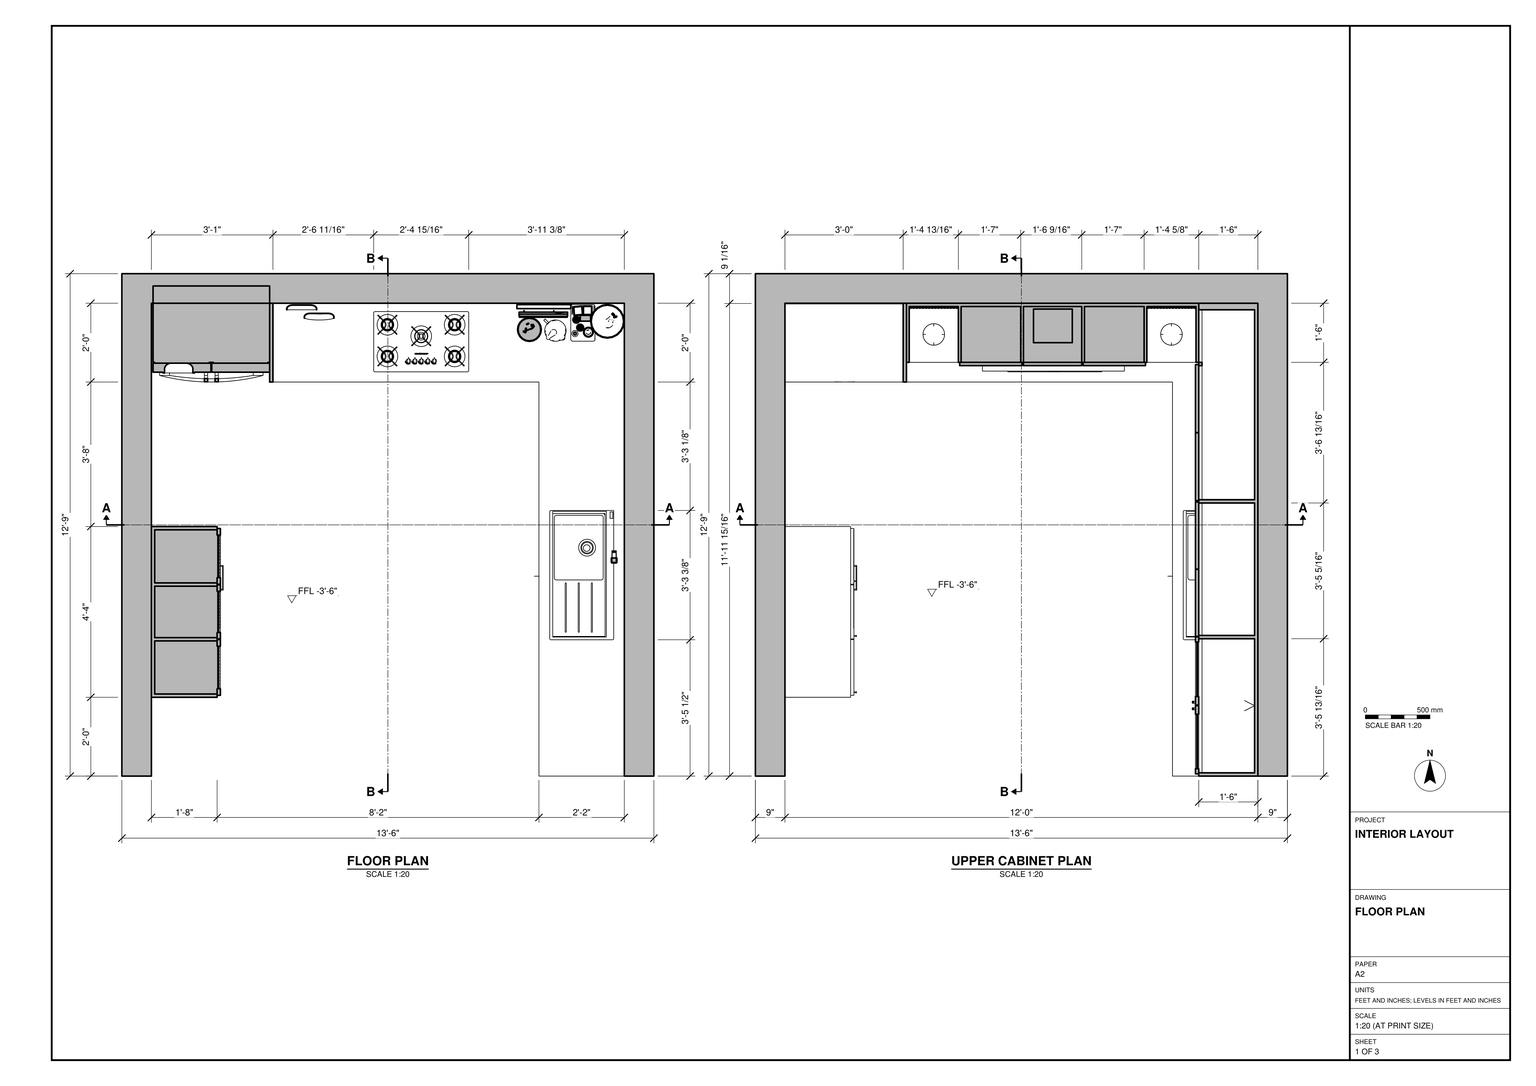
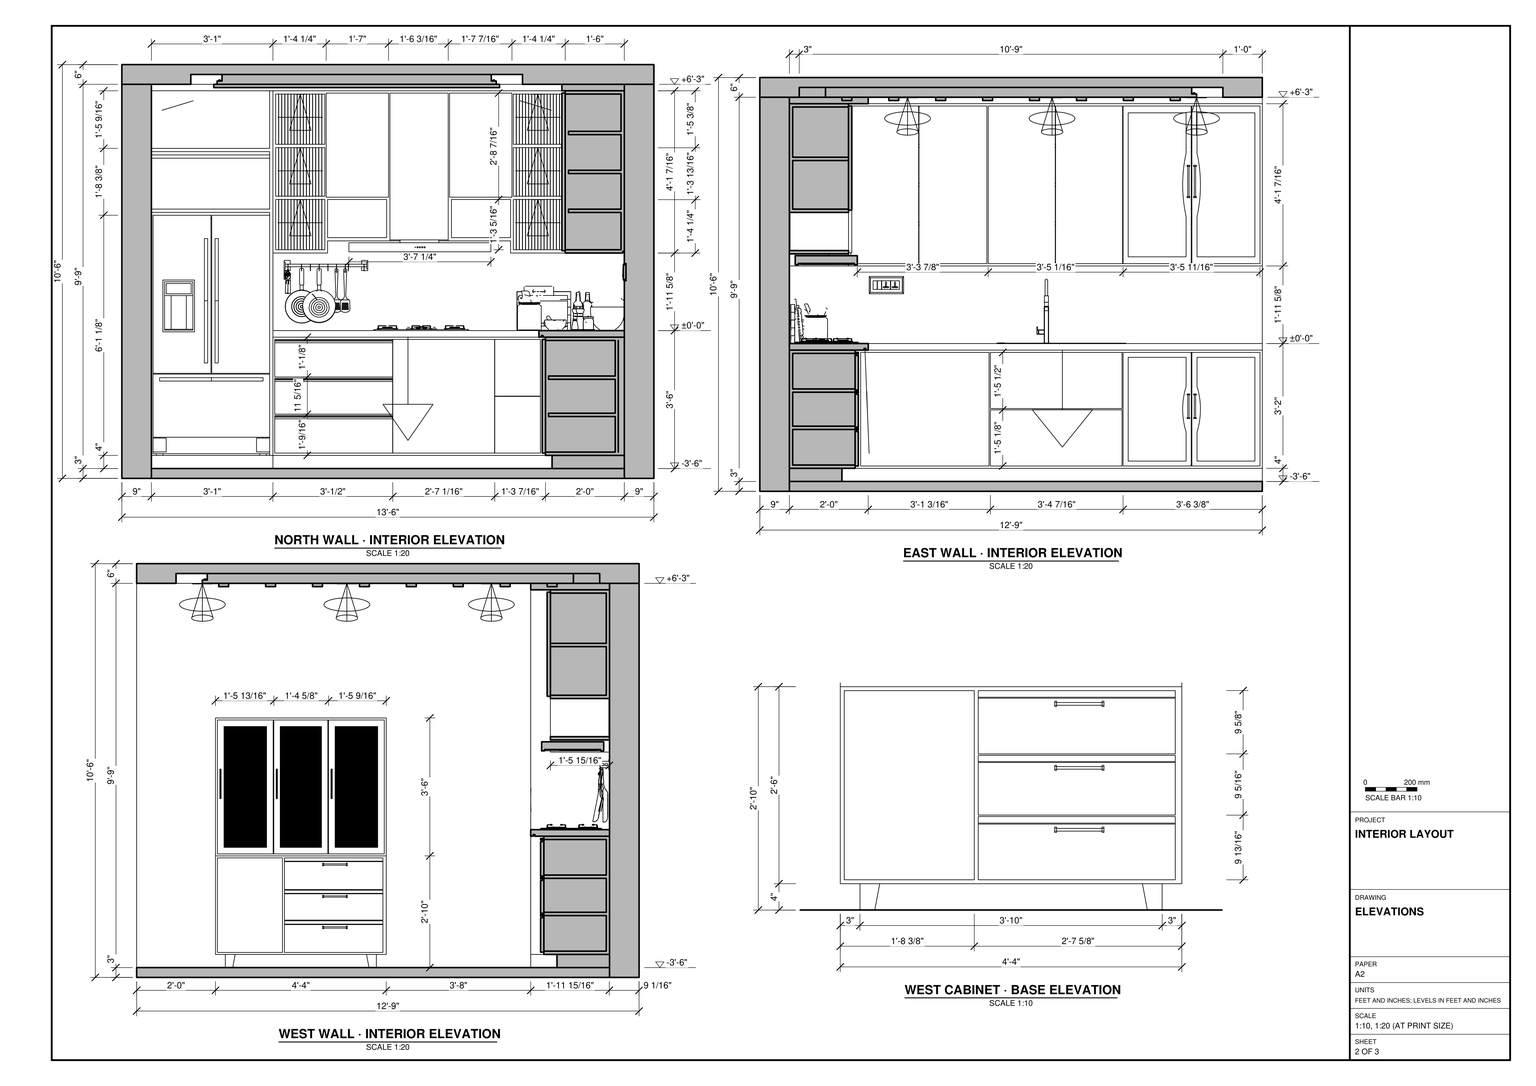
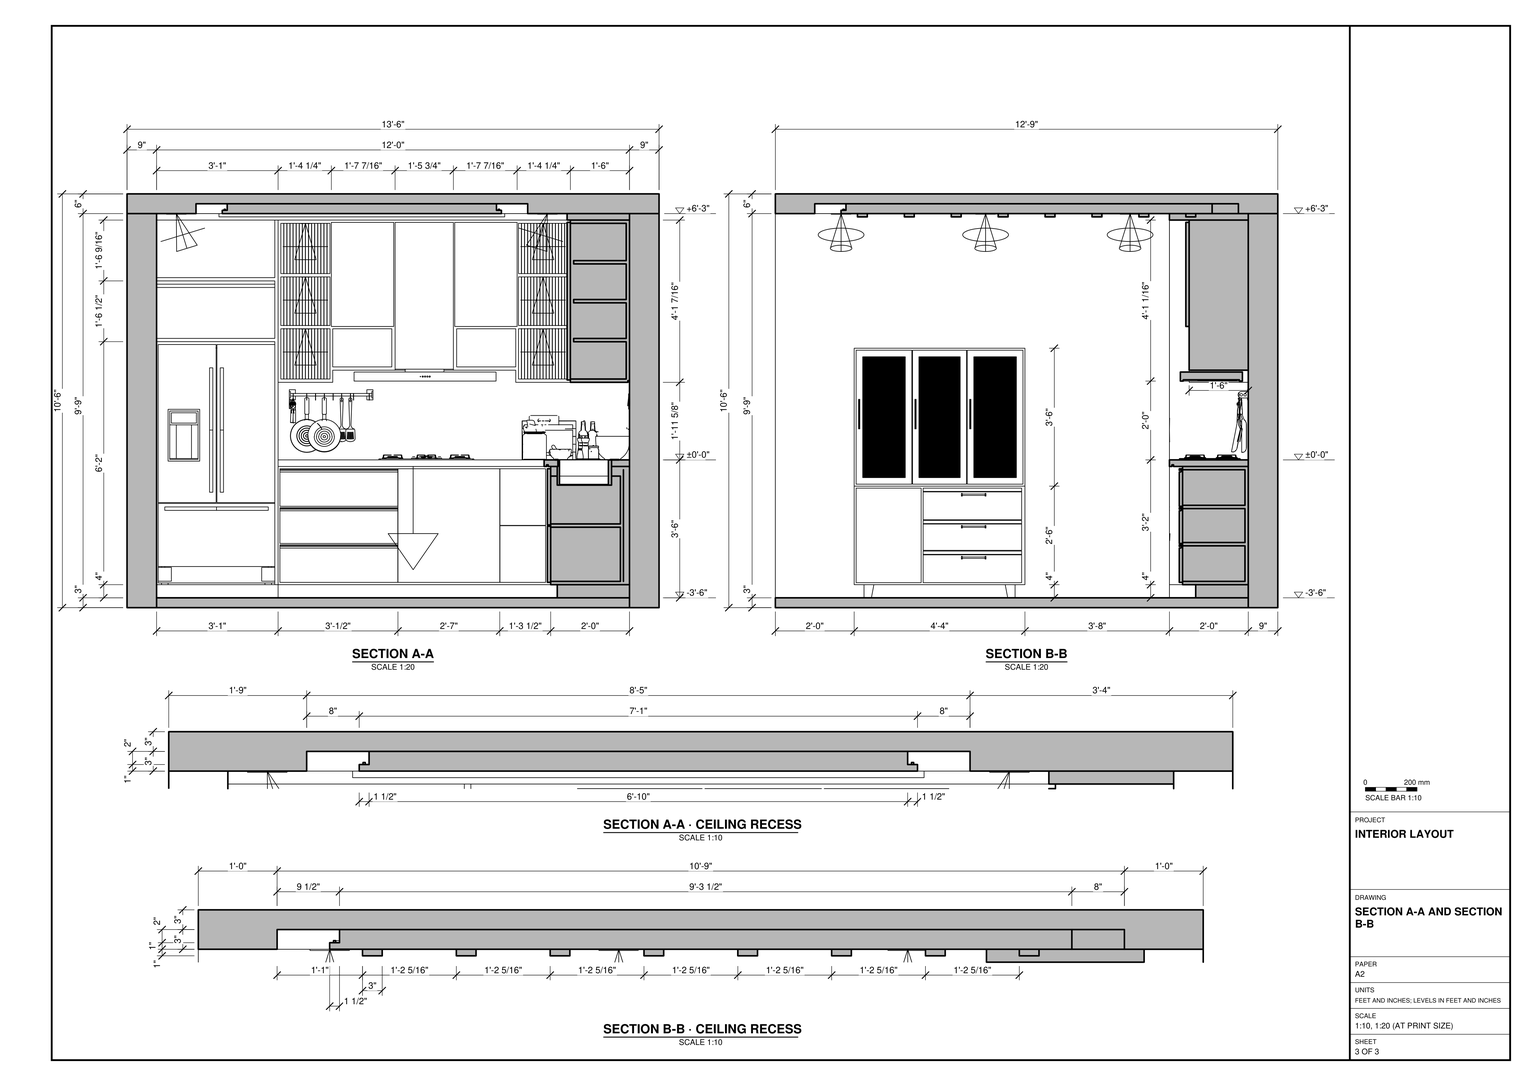
Build the kitchen interior in SketchUp from task_files/diagram_01.pdf. Work in feet and inches. The overall size is 13'-6" east to west by 12'-9" north to south by 10'-6" high. There is one storey at ±0'-0" relative to the ground floor. Use the sections to set heights above the finished floor; the local datum on those sections is at worktop height.

Model the north, east and west walls to their drawn thicknesses, leaving the south side open. Include the floor slab and ceiling. Use both ceiling sections to form the rectangular recess, its inset panel and its stepped edges.

Build the L-shaped worktop and base cabinets along the north and east walls. Place the refrigerator at the west end of the north run, the cooktop beneath the hood, and the sink, drainer and tap on the east return. Use the upper cabinet plan for the cabinet depths and the elevations for the doors, drawer banks, handles and plinths. On the west wall, model the separate storage cabinet with a raised base, drawers and three framed upper doors. Keep the central floor area clear and place the ceiling lights as shown in the elevations.

Decor and loose items, including lamps, appliances and countertop accessories, may be any suitable library components. Keep the walls, slabs, ceiling and each furniture or joinery piece in separate groups or components, and use components for repeated parts. Save one SketchUp model as output_files/fitted_kitchen_with_a_recessed_ceiling.skp.

# SketchUp Ruby script. Lengths in inches.
U = 1.inch
M = Sketchup.active_model
def pt(a) = Geom::Point3d.new(a.map { |v| v * U })
def face(e, loops, mat)
  f = e.add_face(loops[0].map { |a| pt(a) })
  loops[1..].each { |l| e.add_face(l.map { |a| pt(a) }).erase! }
  f.material = f.back_material = mat if mat
  f
end
# faces: each face lists its corners as indices into pts; further lists are holes
def faces(e, pts, list, mat = nil) = list.each { |f| face(e, (f[0].is_a?(Array) ? f : [f]).map { |l| l.map { |i| pts[i] } }, mat) }
# xy, xz, yz: faces in a plane at the given z, y or x. An outline is a flat list of corners, or four numbers for a rectangle; further outlines are holes
def ring(l) = l.size == 4 ? [[l[0], l[1]], [l[2], l[1]], [l[2], l[3]], [l[0], l[3]]] : l.each_slice(2).to_a
def flat(e, list, mat, &to3) = list.each { |f| face(e, (f[0].is_a?(Array) ? f : [f]).map { |l| ring(l).map { |u, v| to3.(u, v) } }, mat) }
def xy(e, z, list, mat = nil) = flat(e, list, mat) { |x, y| [x, y, z] }
def xz(e, y, list, mat = nil) = flat(e, list, mat) { |x, z| [x, y, z] }
def yz(e, x, list, mat = nil) = flat(e, list, mat) { |y, z| [x, y, z] }
def lines(e, pts, list) = list.each { |a, b| e.add_line(pt(pts[a]), pt(pts[b])) }
# prism: a flat outline (further loops are holes) pulled along v
def prism(e, loops, v, mat = nil)
  f = face(e, loops, mat); d = Geom::Vector3d.new(v.map { |x| x * U })
  f.pushpull(f.normal.samedirection?(d) ? d.length : -d.length)
end
def box(e, o, s, mat = nil) = prism(e, [[o, [o[0] + s[0], o[1], o[2]], [o[0] + s[0], o[1] + s[1], o[2]], [o[0], o[1] + s[1], o[2]]]], [0, 0, s[2]], mat)
def at(x, y, z, deg = 0) = Geom::Transformation.translation(pt([x, y, z])) * Geom::Transformation.rotation(ORIGIN, Z_AXIS, deg.degrees)
def axes(o, x, y, z) = Geom::Transformation.new([*x, 0, *y, 0, *z, 0, *pt(o).to_a, 1])
def part(name) = M.definitions.add(name)
# library, detail: a bought-in or finely detailed component or shape, given as its bounding box
def library(name, o, s) = part(name).tap { |d| box(d.entities, o, s) }
def detail(e, o, s) = box(e.add_group.entities, o, s)
def put(e, d, t, mat = nil) = e.add_instance(d, t).tap { |i| i.material = mat if mat }
def group(e, t, mat = nil) = e.add_group.tap { |g| g.transformation = t; g.material = mat if mat }.entities
root = M.entities
M.materials.add("0184 AP 7363 HIGH SPIRITS").color = [199, 226, 231]
M.materials.add("0441 AP 9210 SOFT BLUE").color = [171, 218, 233]
M.materials.add("[Carrera Marble]").color = [207, 207, 207]
M.materials.add("[Marble Carrara Gold Floor Tile]").color = [225, 223, 217]
M.materials.add("[Metal Corrugated Shiny]").color = [232, 207, 153]
M.materials.add("[Stone Marble]").color = [143, 138, 136]
M.materials.add("[Translucent Glass Blue]").color = [154, 179, 222]
M.materials.add("[Wood Cherry Original]").color = [152, 86, 42]
M.materials.add("[Wood Veneer 01]").color = [160, 105, 68]
c1 = part("1")
xy(c1.entities,-0.3,[[-0.45,-1,35.45,0]])
xy(c1.entities,10.13,[[-0.45,-1,35.45,-0.75],[-0.45,-0.75,35.45,-0.72]],"[Metal Corrugated Shiny]")
xy(c1.entities,10.14,[[-0.45,-0.69,35.45,-0.66]],"[Metal Corrugated Shiny]")
xy(c1.entities,10.63,[[-0.45,-1,35.45,-0.97]])
xy(c1.entities,10.65,[[-0.45,-0.92,35.45,-0.9]])
xy(c1.entities,10.88,[[-0.45,-0.75,35.45,-0.72],[-0.45,-0.72,35.45,-0.69]],"[Metal Corrugated Shiny]")
xy(c1.entities,11.13,[[-0.45,-1,35.45,0]],"[Metal Corrugated Shiny]")
xz(c1.entities,-1,[[-0.45,-0.3,35.45,10.13]])
xz(c1.entities,-1,[[-0.45,10.63,35.45,11.13]],"[Metal Corrugated Shiny]")
xz(c1.entities,-0.76,[[-0.45,10.81,35.45,10.83]])
xz(c1.entities,-0.75,[[-0.45,10.86,35.45,10.88]])
xz(c1.entities,-0.39,[[-0.45,10.39,35.45,10.42],[-0.45,10.6,35.45,10.625]],"[Metal Corrugated Shiny]")
xz(c1.entities,-0.375,[[-0.45,10.48,35.45,10.51],[-0.45,10.51,35.45,10.54]],"[Metal Corrugated Shiny]")
xz(c1.entities,0,[[-0.45,-0.3,35.45,11.13]])
yz(c1.entities,-0.45,[[-1,-0.3,-1,10.13,-0.72,10.13,-0.69,10.14,-0.66,10.14,-0.63,10.15,-0.61,10.16,-0.58,10.17,-0.55,10.1875,-0.53,10.2,-0.51,10.22,-0.48,10.24,-0.46,10.26,-0.45,10.29,-0.43,10.3125,-0.42,10.34,-0.4,10.36,-0.39,10.39,-0.39,10.42,-0.38,10.45,-0.375,10.48,-0.375,10.54,-0.38,10.57,-0.39,10.6,-0.39,10.625,-0.4,10.65,-0.42,10.68,-0.43,10.7,-0.45,10.73,-0.46,10.75,-0.48,10.77,-0.51,10.79,-0.53,10.8125,-0.55,10.83,-0.61,10.85,-0.63,10.86,-0.69,10.88,-0.75,10.88,-0.75,10.86,-0.76,10.83,-0.76,10.81,-0.77,10.78,-0.78,10.76,-0.8,10.74,-0.8125,10.72,-0.83,10.7,-0.85,10.68,-0.875,10.67,-0.9,10.65,-0.92,10.65,-0.95,10.64,-0.97,10.63,-1,10.63,-1,11.13,0,11.13,0,-0.3]])
yz(c1.entities,35.45,[[-1,-0.3,0,-0.3,0,11.13,-1,11.13,-1,10.63,-0.97,10.63,-0.95,10.64,-0.92,10.65,-0.9,10.65,-0.875,10.67,-0.85,10.68,-0.83,10.7,-0.8125,10.72,-0.8,10.74,-0.78,10.76,-0.77,10.78,-0.76,10.81,-0.76,10.83,-0.75,10.86,-0.75,10.88,-0.69,10.88,-0.63,10.86,-0.61,10.85,-0.55,10.83,-0.53,10.8125,-0.51,10.79,-0.48,10.77,-0.46,10.75,-0.45,10.73,-0.43,10.7,-0.42,10.68,-0.4,10.65,-0.39,10.625,-0.39,10.6,-0.38,10.57,-0.375,10.54,-0.375,10.48,-0.38,10.45,-0.39,10.42,-0.39,10.39,-0.4,10.36,-0.42,10.34,-0.43,10.3125,-0.45,10.29,-0.46,10.26,-0.48,10.24,-0.51,10.22,-0.53,10.2,-0.55,10.1875,-0.58,10.17,-0.61,10.16,-0.63,10.15,-0.66,10.14,-0.69,10.14,-0.72,10.13,-1,10.13]])
p = [[35.45,-0.66,10.14],[35.45,-0.63,10.15],[-0.45,-0.63,10.15],[-0.45,-0.66,10.14],[35.45,-0.72,10.13],[35.45,-0.69,10.14],
  [-0.45,-0.69,10.14],[-0.45,-0.72,10.13],[35.45,-0.55,10.1875],[35.45,-0.53,10.2],[-0.45,-0.53,10.2],[-0.45,-0.55,10.1875],
  [35.45,-0.58,10.17],[-0.45,-0.58,10.17],[35.45,-0.61,10.16],[-0.45,-0.61,10.16],[35.45,-0.48,10.24],[35.45,-0.46,10.26],
  [-0.45,-0.46,10.26],[-0.45,-0.48,10.24],[35.45,-0.51,10.22],[-0.45,-0.51,10.22],[35.45,-0.45,10.29],[-0.45,-0.45,10.29],
  [35.45,-0.42,10.34],[35.45,-0.4,10.36],[-0.45,-0.4,10.36],[-0.45,-0.42,10.34],[35.45,-0.43,10.3125],[-0.45,-0.43,10.3125],
  [35.45,-0.38,10.45],[35.45,-0.375,10.48],[-0.45,-0.375,10.48],[-0.45,-0.38,10.45],[35.45,-0.39,10.42],[-0.45,-0.39,10.42],
  [35.45,-0.39,10.39],[-0.45,-0.39,10.39],[35.45,-0.375,10.54],[35.45,-0.38,10.57],[-0.45,-0.38,10.57],[-0.45,-0.375,10.54],
  [35.45,-0.95,10.64],[35.45,-0.97,10.63],[-0.45,-0.97,10.63],[-0.45,-0.95,10.64],[35.45,-0.92,10.65],[-0.45,-0.92,10.65],
  [35.45,-0.39,10.625],[35.45,-0.4,10.65],[-0.45,-0.4,10.65],[-0.45,-0.39,10.625],[35.45,-0.39,10.6],[-0.45,-0.39,10.6],
  [35.45,-0.875,10.67],[35.45,-0.9,10.65],[-0.45,-0.9,10.65],[-0.45,-0.875,10.67],[35.45,-0.85,10.68],[-0.45,-0.85,10.68],
  [35.45,-0.83,10.7],[-0.45,-0.83,10.7],[35.45,-0.8125,10.72],[-0.45,-0.8125,10.72],[35.45,-0.8,10.74],[-0.45,-0.8,10.74],
  [35.45,-0.78,10.76],[-0.45,-0.78,10.76],[35.45,-0.45,10.73],[35.45,-0.46,10.75],[-0.45,-0.46,10.75],[-0.45,-0.45,10.73],
  [35.45,-0.43,10.7],[-0.45,-0.43,10.7],[35.45,-0.42,10.68],[-0.45,-0.42,10.68],[35.45,-0.77,10.78],[-0.45,-0.77,10.78],
  [35.45,-0.76,10.81],[-0.45,-0.76,10.81],[35.45,-0.75,10.86],[35.45,-0.76,10.83],[-0.45,-0.76,10.83],[-0.45,-0.75,10.86],
  [35.45,-0.58,10.84],[35.45,-0.61,10.85],[-0.45,-0.61,10.85],[-0.45,-0.58,10.84],[35.45,-0.55,10.83],[-0.45,-0.55,10.83],
  [35.45,-0.53,10.8125],[-0.45,-0.53,10.8125],[35.45,-0.51,10.79],[-0.45,-0.51,10.79],[35.45,-0.48,10.77],[-0.45,-0.48,10.77],
  [35.45,-0.66,10.87],[35.45,-0.69,10.88],[-0.45,-0.69,10.88],[-0.45,-0.66,10.87],[35.45,-0.63,10.86],[-0.45,-0.63,10.86]]
faces(c1.entities,p,[[0,1,2,3],[4,5,6,7],[8,9,10,11],[12,8,11,13],[14,12,13,15],[1,14,15,2],[16,17,18,19],[20,16,19,21],
  [9,20,21,10],[17,22,23,18],[24,25,26,27],[28,24,27,29],[22,28,29,23],[30,31,32,33],[34,30,33,35],[25,36,37,26],
  [38,39,40,41],[48,49,50,51],[39,52,53,40],[68,69,70,71],[72,68,71,73],[74,72,73,75],[49,74,75,50],[84,85,86,87],
  [88,84,87,89],[90,88,89,91],[92,90,91,93],[94,92,93,95],[69,94,95,70],[96,97,98,99],[100,96,99,101],[85,100,101,86]],"[Metal Corrugated Shiny]")
faces(c1.entities,p,[[42,43,44,45],[46,42,45,47],[54,55,56,57],[58,54,57,59],[60,58,59,61],[62,60,61,63],[64,62,63,65],[66,64,65,67],
  [76,66,67,77],[78,76,77,79],[80,81,82,83]])
c2 = part("2")
box(c2.entities,[-1,-0.3,-0.3],[1,40.1,17.1])
c3 = part("3")
box(c3.entities,[-20,0,0],[20,41,0.39])
c4 = part("Group156\#1")
p = [[0,0,0],[0,0,-10.12],[-5.02,0,-10.12],[32.7,-0.05,0],[-32.7,-0.05,0],[32.7,0.05,0],
  [32.7,0,0],[-32.7,0.05,0],[5.02,0,-10.12],[-32.7,0,0],[0,0,-16.375]]
lines(c4.entities,p,[[0,1],[1,2],[3,4],[5,6],[7,5],[1,8],[9,0],[0,6],[8,10],[4,9],[6,3],[2,10],
  [9,7]])
c5 = part("Rectangle Light")
put(c5.entities,c4,at(0,0,0))
c6 = part("5")
xy(c6.entities,-0.61,[[-17,0.0625,-16,40.83]])
xy(c6.entities,-0.44,[[-16.3125,0.0625,-16,40.83]])
xy(c6.entities,-0.11,[[-16.3125,0.0625,-16,40.83]])
xy(c6.entities,0,[[-16,0,0,40.83]],"[Translucent Glass Blue]")
xy(c6.entities,0.39,[[-17,0.0625,-16,40.83]])
xy(c6.entities,0.39,[[-16,0,0,40.83]],"[Translucent Glass Blue]")
xz(c6.entities,0,[[-16,0,0,0.39]],"[Translucent Glass Blue]")
xz(c6.entities,0.0625,[[-17,-0.61,-16,-0.61,-16,-0.44,-16.3125,-0.44,-16.3125,-0.11,-16,-0.11,-16,0.39,-17,0.39]])
xz(c6.entities,40.83,[[-16,0,0,0.39]],"[Translucent Glass Blue]")
yz(c6.entities,-17,[[0.0625,-0.61,40.83,0.39]])
yz(c6.entities,-16.3125,[[0.0625,-0.44,40.83,-0.11]])
yz(c6.entities,-16,[[0.0625,-0.61,40.83,-0.44],[0.0625,-0.11,40.83,0],[0.0625,0,40.83,0.39]])
yz(c6.entities,-16,[[0,0,0.0625,0.39]],"[Translucent Glass Blue]")
yz(c6.entities,0,[[0,0,40.83,0.39]],"[Translucent Glass Blue]")
put(c6.entities,c5,axes([-16.03,20.45,-0.19],[0,0.62341,0],[-0.20108,0,-0.97958],[-0.97958,0,0.20108]))
g1 = group(c6.entities,at(-16.3125,0.0625,-0.27))
box(g1,[0,0,0],[0.25,40.77,0.17])
c7 = library("Rangemaaster flat hood",[-3.82,0.71,0],[43.23,19.01,40.35])
c8 = library("French door refrigerator",[0,0,0],[35.5,29.25,69.5])
c9 = part("POI-E1497-320-1917\#1")
xy(c9.entities,0,[[0,0,0.29,0.83],[7.21,0,7.5,0.83]])
xy(c9.entities,0.64,[[0.29,0.21,7.21,0.62]])
xy(c9.entities,0.875,[[0,0.21,7.5,0.62]])
xz(c9.entities,0.21,[[0,0.64,7.5,0.875]])
xz(c9.entities,0.62,[[0,0.64,7.5,0.875]])
yz(c9.entities,0,[[0,0,0.21,0.64,0.21,0.875,0.62,0.875,0.62,0.64,0.83,0]])
yz(c9.entities,0.29,[[0,0,0.83,0,0.62,0.64,0.21,0.64]])
yz(c9.entities,7.21,[[0,0,0.21,0.64,0.62,0.64,0.83,0]])
yz(c9.entities,7.5,[[0,0,0.83,0,0.62,0.64,0.62,0.875,0.21,0.875,0.21,0.64]])
p = [[0,0.21,0.64],[0,0,0],[0.29,0,0],[0.29,0.21,0.64],[7.21,0.21,0.64],[7.21,0,0],
  [7.5,0,0],[7.5,0.21,0.64],[0,0.83,0],[0,0.62,0.64],[0.29,0.62,0.64],[0.29,0.83,0],
  [7.5,0.83,0],[7.5,0.62,0.64],[7.21,0.62,0.64],[7.21,0.83,0]]
faces(c9.entities,p,[[0,1,2,3],[4,5,6,7],[8,9,10,11],[12,13,14,15]])
c10 = library("kitchen utensil",[-39.88,-27.4,0],[79.77,28.4,32.96])
c11 = library("Cookware hanging rail",[-2.09,-19.1875,0],[25.71,19.1875,6.07])
c12 = library("9",[-6.9,-3.96,-12.62],[16.56,13.95,14.65])
c13 = library("switch board",[0,0,0],[0.88,10.49,5.27])
c14 = library("Group\#1",[0,0,0],[162,153,126])
c15 = library("Group\#7",[0,0,-31.45],[107,144,53.06])
c16 = library("Group\#26",[0,0,0],[28.9375,18.36,1.53])
c17 = library("Group\#14",[0,0,0],[107,144,49.41])
xy(root,3,[[122,0,144,128],[0,120,0,144,144,144,144,128,37,128,37,120]])
xy(root,7,[[122,0,144,128],[0,120,36,144],[36,120,37,144],[37,128,144,144]])
xy(root,81,[[0,120,36,143.92]],"[Wood Cherry Original]")
xy(root,82,[[0,120,36,143.92]],"[Wood Cherry Original]")
xy(root,99.5,[[0,120,36,143.92]],"[Wood Cherry Original]")
xy(root,100.5,[[0,120,36,143.92]],"[Wood Cherry Original]")
xy(root,118.03,[[125,0,144,120],[0,120,36,143.92],[36,120,37,144],[37,120,144,144]])
xy(root,120,[[125,0,144,0,144,144,0,144,0,120,125,120]])
xz(root,0,[[122,3,144,7],[125,118.03,144,120]])
xz(root,120,[[0,118.03,125,120]])
xz(root,120,[[0,3,37,7]],"[Carrera Marble]")
xz(root,120,[[36,7,37,7,37,118.03,36,118.03,36,100.5,0,100.5,0,99.5,36,99.5,36,82,0,82,0,81,36,81]],"[Wood Veneer 01]")
xz(root,128,[[122,3,144,7]])
xz(root,128,[[37,3,122,7]],"[Carrera Marble]")
xz(root,143.92,[[0,81,36,82],[0,99.5,36,100.5]],"[Wood Cherry Original]")
xz(root,143.92,[[0,82,36,99.5],[0,100.5,36,118.03]],"[Wood Veneer 01]")
xz(root,144,[[0,3,144,7],[36,7,37,7,37,118.03,36,118.03,36,98.5,0,98.5,0,97.5,36,97.5]])
xz(root,144,[[0,98.5,36,118.03]],"[Wood Veneer 01]")
yz(root,0,[[120,3,144,7],[120,81,143.92,82],[143.92,97.5,144,98.5],[120,99.5,143.92,100.5],[120,118.03,144,120]])
yz(root,0,[[143.92,76,144,97.5],[143.92,98.5,144,118.03]],"[Wood Veneer 01]")
yz(root,36,[[120,7,120,81,143.92,81,143.92,76,144,76,144,7]],"[Wood Cherry Original]")
yz(root,36,[[143.92,76,144,97.5],[120,82,143.92,99.5],[143.92,98.5,144,118.03],[120,100.5,143.92,118.03]],"[Wood Veneer 01]")
yz(root,37,[[120,3,128,7]],"[Carrera Marble]")
yz(root,37,[[120,7,144,118.03]],"[Wood Veneer 01]")
yz(root,122,[[0,3,128,7]],"[Carrera Marble]")
yz(root,125,[[0,118.03,120,120]])
yz(root,144,[[0,3,128,7],[128,3,144,7],[120,118.03,144,120]])
# 2 loose lines left out
put(root,c1,at(38,124,31.17),"0441 AP 9210 SOFT BLUE")
put(root,c1,axes([38,124,19.83],[1,0,0],[0,1,0],[0,0,0.95385]),"0441 AP 9210 SOFT BLUE")
put(root,c1,at(38,124,8),"0441 AP 9210 SOFT BLUE")
put(root,c2,at(120,43,25.5),"0441 AP 9210 SOFT BLUE")
put(root,c2,at(120,43,8),"0441 AP 9210 SOFT BLUE")
put(root,c3,at(141,1,19.2),"[Translucent Glass Blue]")
put(root,c3,at(141,1,30.4),"[Translucent Glass Blue]")
put(root,c6,at(143,1,83.34))
put(root,c6,at(143,1,95.1))
put(root,c6,at(143,1,106.85))
put(root,c7,at(63.95,122.5,69))
put(root,c8,axes([36,149.25,7],[-1,0,0],[0,-1,0],[0,0,1.05223]))
put(root,c9,axes([119,22.08,22.14],[0,0,1],[0,1,0],[-1,0,0]))
put(root,c9,axes([119,20.92,22.14],[0,0,1],[0,-1,0],[-1,0,0]))
put(root,c9,axes([125,22.08,89.4],[0,0,1.3189],[0,1,0],[-1,0,0]))
put(root,c9,axes([125,20.92,89.4],[0,0,1.3189],[0,-1,0],[-1,0,0]))
put(root,c10,axes([127.65,143.59,45],[0.41,0,0],[0,0.41,0],[0,0,0.41]))
put(root,c11,axes([42.26,144,66.375],[1,0,0],[0,0,1],[0,-1,0]))
put(root,c12,at(116,17,120))
put(root,c12,at(116,61,120))
put(root,c12,at(116,105,120))
put(root,c12,axes([9,17,120],[-1,0,0],[0,1,0],[0,0,1]))
put(root,c12,axes([9,61,120],[-1,0,0],[0,1,0],[0,0,1]))
put(root,c12,axes([9,105,120],[-1,0,0],[0,1,0],[0,0,1]))
put(root,c13,at(144.29,119.7,60.16,180))
put(root,c14,at(-9,0,0))
g2 = group(root,at(0,0,0))
xy(g2,0,[[0,0,144,144]])
xy(g2,3,[[122,0,144,0,144,144,0,144,0,120,37,120,37,128,122,128]])
xy(g2,3,[[0,0,122,0,122,128,37,128,37,120,0,120]],"[Marble Carrara Gold Floor Tile]")
xz(g2,0,[[0,0,144,3]])
xz(g2,144,[[0,0,144,3]])
yz(g2,0,[[0,0,144,3]])
yz(g2,144,[[0,0,144,3]])
g3 = group(root,at(74,124,8),"0441 AP 9210 SOFT BLUE")
box(g3,[-0.5,-1,-0.3],[31,1,34.6])
g4 = group(root,at(105,124,8),"0441 AP 9210 SOFT BLUE")
box(g4,[-0.45,-1,17.05],[13.9,1,17.25])
box(g4,[-0.45,-1,-0.3],[13.9,1,17.25])
put(root,c15,at(37,0,43),"[Stone Marble]")
g5 = group(root,at(37,144,7),"0184 AP 7363 HIGH SPIRITS")
xy(g5,0,[[0,-20,83,0]])
xy(g5,1,[[1,-20,36,-1],[37,-20,67,-1],[68,-20,80,-1]])
xy(g5,11.83,[[1,-20,36,-1]])
xy(g5,12.83,[[1,-20,36,-1]])
xy(g5,17.5,[[68,-20,80,-1]])
xy(g5,18.5,[[68,-20,80,-1]])
xy(g5,23.17,[[1,-20,36,-1]])
xy(g5,24.17,[[1,-20,36,-1]])
xy(g5,35,[[1,-20,36,-1],[37,-20,67,-1],[68,-20,80,-1]])
xy(g5,36,[[0,-20,83,0]])
xz(g5,-20,[[[0,0,83,36],[37,1,67,35],[1,1,36,11.83],[1,24.17,36,35],[1,12.83,36,23.17],[68,18.5,80,35],[68,1,80,17.5]]])
xz(g5,-1,[[1,1,36,11.83],[37,1,67,35],[68,1,80,17.5],[1,12.83,36,23.17],[68,18.5,80,35],
  [1,24.17,36,35]])
xz(g5,0,[[0,0,83,36]])
yz(g5,0,[[-20,0,0,36]])
yz(g5,1,[[-20,1,-1,11.83],[-20,12.83,-1,23.17],[-20,24.17,-1,35]])
yz(g5,36,[[-20,1,-1,11.83],[-20,12.83,-1,23.17],[-20,24.17,-1,35]])
yz(g5,37,[[-20,1,-1,35]])
yz(g5,67,[[-20,1,-1,35]])
yz(g5,68,[[-20,1,-1,17.5],[-20,18.5,-1,35]])
yz(g5,80,[[-20,1,-1,17.5],[-20,18.5,-1,35]])
yz(g5,83,[[-20,0,0,36]])
g6 = group(root,at(120,83.5,8),"0441 AP 9210 SOFT BLUE")
box(g6,[-1,-0.3,-0.3],[1,39.1,34.6])
g7 = group(root,at(120,1,8),"0441 AP 9210 SOFT BLUE")
xy(g7,-0.3,[[-1,-0.3125,0,20.4375],[-1,20.64,0,41.39]])
xy(g7,1.2,[[-1,1.25,0,18.875],[-1,22.2,0,39.83]])
xy(g7,32.8,[[-1,1.25,0,18.875],[-1,22.2,0,39.83]])
xy(g7,34.3,[[-1,-0.3125,0,20.4375],[-1,20.64,0,41.39]])
xz(g7,-0.3125,[[-1,-0.3,0,34.3]])
xz(g7,1.25,[[-1,1.2,0,32.8]])
xz(g7,18.875,[[-1,1.2,0,10.11],[-1,23.89,0,32.8]])
xz(g7,20.4375,[[-1,-0.3,0,34.3]])
xz(g7,20.64,[[-1,-0.3,0,34.3]])
xz(g7,22.2,[[-1,1.2,0,10.11],[-1,23.89,0,32.8]])
xz(g7,39.83,[[-1,1.2,0,32.8]])
xz(g7,41.39,[[-1,-0.3,0,34.3]])
yz(g7,-1,[[[-0.3125,-0.3,20.4375,34.3],[1.25,1.2,18.875,1.2,18.875,10.11,18.67,10.78,18.49,11.46,18.34,12.14,18.21,12.83,18.09,13.52,18,14.21,17.93,14.91,17.88,15.6,17.85,16.3,17.84,17,17.85,17.7,17.88,18.4,17.93,19.09,18,19.79,18.09,20.48,18.21,21.17,18.34,21.86,18.49,22.54,18.67,23.22,18.875,23.89,18.875,32.8,1.25,32.8]],[[20.64,-0.3,41.39,34.3],[22.2,1.2,39.83,1.2,39.83,32.8,22.2,32.8,22.2,23.89,22.41,23.22,22.59,22.54,22.74,21.86,22.87,21.17,22.99,20.48,23.08,19.79,23.15,19.09,23.2,18.4,23.23,17.7,23.24,17,23.23,16.3,23.2,15.6,23.15,14.91,23.08,14.21,22.99,13.52,22.87,12.83,22.74,12.14,22.59,11.46,22.41,10.78,22.2,10.11]]])
yz(g7,0,[[[-0.3125,-0.3,20.4375,34.3],[1.25,1.2,1.25,32.8,18.875,32.8,18.875,23.89,18.67,23.22,18.49,22.54,18.34,21.86,18.21,21.17,18.09,20.48,18,19.79,17.93,19.09,17.88,18.4,17.85,17.7,17.84,17,17.85,16.3,17.88,15.6,17.93,14.91,18,14.21,18.09,13.52,18.21,12.83,18.34,12.14,18.49,11.46,18.67,10.78,18.875,10.11,18.875,1.2]],[20.4375,-0.3,20.64,34.3],[[20.64,-0.3,41.39,34.3],[22.2,1.2,22.2,10.11,22.41,10.78,22.59,11.46,22.74,12.14,22.87,12.83,22.99,13.52,23.08,14.21,23.15,14.91,23.2,15.6,23.23,16.3,23.24,17,23.23,17.7,23.2,18.4,23.15,19.09,23.08,19.79,22.99,20.48,22.87,21.17,22.74,21.86,22.59,22.54,22.41,23.22,22.2,23.89,22.2,32.8,39.83,32.8,39.83,1.2]]])
p = [[-1,18.67,10.78],[-1,18.875,10.11],[0,18.875,10.11],[0,18.67,10.78],[-1,22.2,10.11],[-1,22.41,10.78],
  [0,22.41,10.78],[0,22.2,10.11],[-1,18.49,11.46],[0,18.49,11.46],[-1,22.59,11.46],[0,22.59,11.46],
  [-1,18.34,12.14],[0,18.34,12.14],[-1,22.74,12.14],[0,22.74,12.14],[-1,18.21,12.83],[0,18.21,12.83],
  [-1,22.87,12.83],[0,22.87,12.83],[-1,18.09,13.52],[0,18.09,13.52],[-1,22.99,13.52],[0,22.99,13.52],
  [-1,18,14.21],[0,18,14.21],[-1,23.08,14.21],[0,23.08,14.21],[-1,17.93,14.91],[0,17.93,14.91],
  [-1,23.15,14.91],[0,23.15,14.91],[-1,17.88,15.6],[0,17.88,15.6],[-1,23.2,15.6],[0,23.2,15.6],
  [-1,17.85,16.3],[0,17.85,16.3],[-1,23.23,16.3],[0,23.23,16.3],[-1,17.84,17],[0,17.84,17],
  [-1,23.24,17],[0,23.24,17],[-1,17.85,17.7],[0,17.85,17.7],[-1,23.23,17.7],[0,23.23,17.7],
  [-1,17.88,18.4],[0,17.88,18.4],[-1,23.2,18.4],[0,23.2,18.4],[-1,17.93,19.09],[0,17.93,19.09],
  [-1,23.15,19.09],[0,23.15,19.09],[-1,18,19.79],[0,18,19.79],[-1,23.08,19.79],[0,23.08,19.79],
  [-1,18.09,20.48],[0,18.09,20.48],[-1,22.99,20.48],[0,22.99,20.48],[-1,18.21,21.17],[0,18.21,21.17],
  [-1,22.87,21.17],[0,22.87,21.17],[-1,18.34,21.86],[0,18.34,21.86],[-1,22.74,21.86],[0,22.74,21.86],
  [-1,18.49,22.54],[0,18.49,22.54],[-1,22.59,22.54],[0,22.59,22.54],[-1,18.67,23.22],[0,18.67,23.22],
  [-1,22.41,23.22],[0,22.41,23.22],[-1,18.875,23.89],[0,18.875,23.89],[-1,22.2,23.89],[0,22.2,23.89]]
faces(g7,p,[[0,1,2,3],[4,5,6,7],[8,0,3,9],[5,10,11,6],[12,8,9,13],[10,14,15,11],[16,12,13,17],[14,18,19,15],
  [20,16,17,21],[18,22,23,19],[24,20,21,25],[22,26,27,23],[28,24,25,29],[26,30,31,27],[32,28,29,33],[30,34,35,31],
  [36,32,33,37],[34,38,39,35],[40,36,37,41],[38,42,43,39],[44,40,41,45],[42,46,47,43],[48,44,45,49],[46,50,51,47],
  [52,48,49,53],[50,54,55,51],[56,52,53,57],[54,58,59,55],[60,56,57,61],[58,62,63,59],[64,60,61,65],[62,66,67,63],
  [68,64,65,69],[66,70,71,67],[72,68,69,73],[70,74,75,71],[76,72,73,77],[74,78,79,75],[80,76,77,81],[78,82,83,79]])
g8 = group(g7,at(-0.375,1.25,1.2),"[Translucent Glass Blue]")
prism(g8,[[[0,38.58,31.6],[0,20.96,31.6],[0,20.96,22.69],[0,21.16,22.02],[0,21.34,21.34],[0,21.49,20.66],[0,21.625,19.97],[0,21.74,19.28],[0,21.83,18.59],[0,21.9,17.89],[0,21.95,17.2],[0,21.99,16.5],[0,22,15.8],[0,21.99,15.1],[0,21.95,14.4],[0,21.9,13.71],[0,21.83,13.01],[0,21.74,12.32],[0,21.625,11.625],[0,21.49,10.9375],[0,21.34,10.26],[0,21.16,9.58],[0,20.96,8.91],[0,20.96,0],[0,38.58,0]]],[-0.2,0,0])
prism(g8,[[[0,17.63,31.6],[0,0,31.6],[0,0,0],[0,17.63,0],[0,17.63,8.91],[0,17.42,9.58],[0,17.25,10.26],[0,17.09,10.9375],[0,16.96,11.625],[0,16.85,12.32],[0,16.75,13.01],[0,16.68,13.71],[0,16.63,14.4],[0,16.6,15.1],[0,16.59,15.8],[0,16.6,16.5],[0,16.63,17.2],[0,16.68,17.89],[0,16.75,18.59],[0,16.85,19.28],[0,16.96,19.97],[0,17.09,20.66],[0,17.25,21.34],[0,17.42,22.02],[0,17.63,22.69]]],[-0.2,0,0])
g9 = group(root,at(144,0,7),"0184 AP 7363 HIGH SPIRITS")
xy(g9,0,[[-24,0,0,128],[-24,128,0,144]])
xy(g9,1,[[-24,1,-2.77,42],[-24,43,-2.77,82.5],[-24,83.5,-2.77,83.5,-2.77,143,-23.08,143,-23.08,122,-24,122]])
xy(g9,11.83,[[-23.08,83.5,-2.77,143]])
xy(g9,12.83,[[-23.08,83.5,-2.77,143]])
xy(g9,17.5,[[-24,43,-2.77,82.5]])
xy(g9,18.5,[[-24,43,-2.77,82.5]])
xy(g9,23.17,[[-23.08,83.5,-2.77,143]])
xy(g9,24.17,[[-23.08,83.5,-2.77,143]])
xy(g9,30.3125,[[-22,43,-5.47,43,-5.47,79.65,-22,79.57]])
xy(g9,33.0625,[[-22,42.27,-5.47,42.35,-5.47,43,-22,43],[-24,43,-24,82.5,-2.77,82.5,-2.77,43,-5.47,43,-5.47,79.65,-22,79.57,-22,43]])
xy(g9,35,[[-24,1,-2.77,42],[-24,83.5,-24,122,-23.08,122,-23.08,143,-2.77,143,-2.77,83.5]])
xy(g9,36,[[[-24,0,0,144],[-22,42.27,-22,80.625,-5.47,80.71,-5.47,42.35]]])
xz(g9,0,[[-24,0,0,36]])
xz(g9,1,[[-24,1,-2.77,35]])
xz(g9,42,[[-24,1,-2.77,35]])
xz(g9,43,[[-24,1,-2.77,17.5],[-24,18.5,-24,33.0625,-22,33.0625,-22,30.3125,-5.47,30.3125,-5.47,33.0625,-2.77,33.0625,-2.77,18.5],[-22,30.3125,-5.47,33.0625]])
xz(g9,82.5,[[-24,1,-2.77,17.5],[-24,18.5,-2.77,33.0625]])
xz(g9,83.5,[[-24,1,-24,35,-2.77,35,-2.77,24.17,-23.08,24.17,-23.08,23.17,-2.77,23.17,-2.77,12.83,-23.08,12.83,-23.08,11.83,-2.77,11.83,-2.77,1]])
xz(g9,122,[[-24,1,-23.08,35]])
xz(g9,143,[[-24,1,-23.08,35],[-2.77,1,-1.85,1,-1.85,35,-2.77,35,-2.77,24.17,-23.08,24.17,-23.08,23.17,-2.77,23.17,-2.77,12.83,-23.08,12.83,-23.08,11.83,-2.77,11.83],[-23.08,1,-2.77,11.83],[-23.08,12.83,-2.77,23.17],[-23.08,24.17,-2.77,35]])
xz(g9,144,[[-24,0,0,36]])
yz(g9,-24,[[[0,0,144,36],[1,1,42,35],[83.5,1,122,35],[43,1,82.5,17.5],[124,1,143,35],[43,18.5,82.5,33.0625]]])
yz(g9,-23.08,[[122,1,143,11.83],[83.5,11.83,122,12.83],[122,11.83,143,12.83],[122,12.83,143,23.17],[83.5,23.17,122,24.17],
  [122,23.17,143,24.17],[122,24.17,143,35]])
yz(g9,-22,[[43,30.3125,79.57,33.0625],[42.27,33.0625,79.57,33.0625,80.625,36,42.27,36]])
yz(g9,-5.47,[[43,30.3125,79.65,33.0625],[42.35,33.0625,42.35,36,80.71,36,79.65,33.0625]])
yz(g9,-2.77,[[1,1,42,35],[43,1,82.5,17.5],[83.5,1,143,11.83],[83.5,12.83,143,23.17],[43,18.5,82.5,33.0625],
  [83.5,24.17,143,35]])
yz(g9,-1.85,[[43,1,143,35]])
yz(g9,0,[[0,0,144,36]])
# 4 loose lines left out
p = [[-5.47,79.65,33.0625],[-22,79.57,33.0625],[-22,79.57,30.3125],[-5.47,79.65,30.3125],[-22,42.27,36],[-5.47,42.35,36],
  [-5.47,42.35,33.0625],[-22,42.27,33.0625],[-5.47,80.71,36],[-22,80.625,36]]
faces(g9,p,[[0,1,2,3],[4,5,6,7],[8,9,1,0]])
put(root,c16,at(67.6875,123.1,45))
put(root,c17,at(37,0,68.62),"0184 AP 7363 HIGH SPIRITS")
